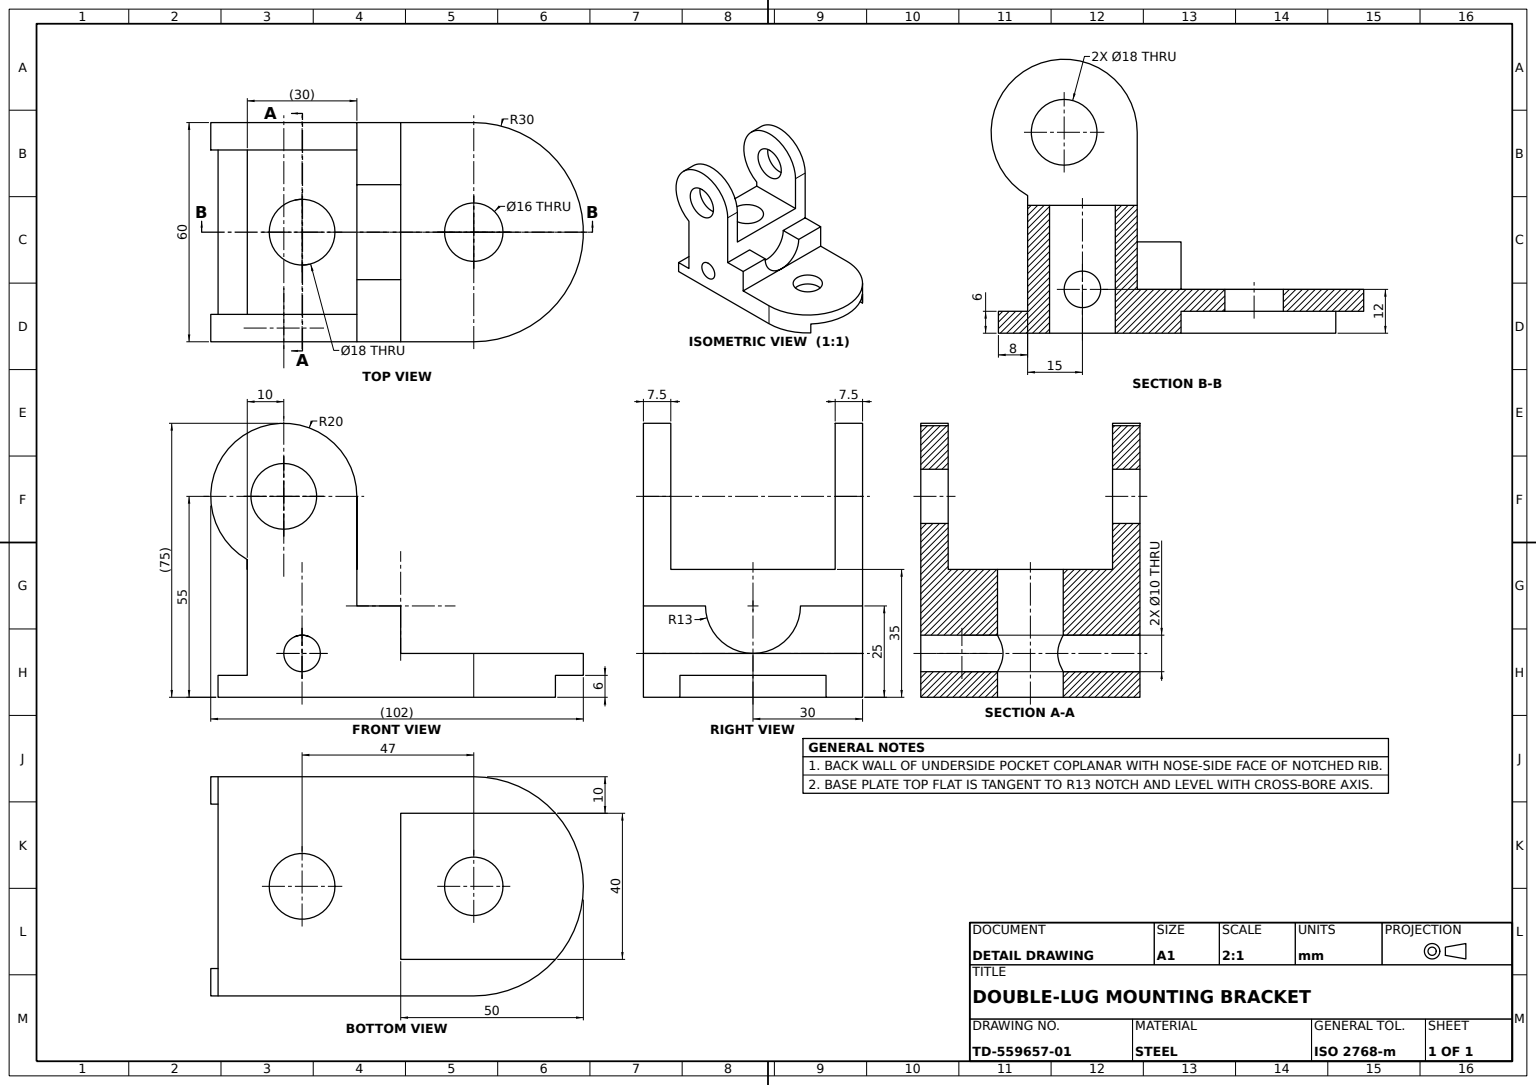
ISO-10303-21;
HEADER;
FILE_DESCRIPTION((''),'2;1');
FILE_NAME('','',(''),(''),'','','');
FILE_SCHEMA(('AUTOMOTIVE_DESIGN'));
ENDSEC;
DATA;
#1=APPLICATION_CONTEXT('');
#2=PRODUCT_CONTEXT('',#1,'mechanical');
#3=PRODUCT('','','',(#2));
#4=PRODUCT_DEFINITION_FORMATION('','',#3);
#5=PRODUCT_DEFINITION_CONTEXT('',#1,'design');
#6=PRODUCT_DEFINITION('','',#4,#5);
#7=PRODUCT_DEFINITION_SHAPE('','',#6);
#8=(LENGTH_UNIT()NAMED_UNIT(*)SI_UNIT(.MILLI.,.METRE.));
#9=(NAMED_UNIT(*)PLANE_ANGLE_UNIT()SI_UNIT($,.RADIAN.));
#10=(NAMED_UNIT(*)SI_UNIT($,.STERADIAN.)SOLID_ANGLE_UNIT());
#11=UNCERTAINTY_MEASURE_WITH_UNIT(LENGTH_MEASURE(0.005),#8,'distance_accuracy_value','');
#12=(GEOMETRIC_REPRESENTATION_CONTEXT(3)GLOBAL_UNCERTAINTY_ASSIGNED_CONTEXT((#11))GLOBAL_UNIT_ASSIGNED_CONTEXT((#8,#9,#10))REPRESENTATION_CONTEXT('',''));
#13=CARTESIAN_POINT('',(12.,0.,12.));
#14=VERTEX_POINT('',#13);
#15=CARTESIAN_POINT('',(20.,0.,12.));
#16=DIRECTION('',(0.,0.,-1.));
#17=DIRECTION('',(-1.,0.,0.));
#18=AXIS2_PLACEMENT_3D('',#15,#16,#17);
#19=CIRCLE('',#18,8.);
#20=EDGE_CURVE('',#14,#14,#19,.T.);
#21=ORIENTED_EDGE('',*,*,#20,.T.);
#22=EDGE_LOOP('',(#21));
#23=FACE_BOUND('',#22,.T.);
#24=CARTESIAN_POINT('',(0.,-30.,12.));
#25=VERTEX_POINT('',#24);
#26=CARTESIAN_POINT('',(0.,0.,12.));
#27=VERTEX_POINT('',#26);
#28=DIRECTION('',(0.,1.,0.));
#29=VECTOR('',#28,1000.);
#30=LINE('',#24,#29);
#31=EDGE_CURVE('',#25,#27,#30,.T.);
#32=ORIENTED_EDGE('',*,*,#31,.F.);
#33=CARTESIAN_POINT('',(20.,-30.,12.));
#34=VERTEX_POINT('',#33);
#35=CARTESIAN_POINT('',(-50.,-30.,12.));
#36=DIRECTION('',(1.,0.,0.));
#37=VECTOR('',#36,1000.);
#38=LINE('',#35,#37);
#39=EDGE_CURVE('',#25,#34,#38,.T.);
#40=ORIENTED_EDGE('',*,*,#39,.T.);
#41=CARTESIAN_POINT('',(20.,30.,12.));
#42=VERTEX_POINT('',#41);
#43=DIRECTION('',(0.,0.,1.));
#44=AXIS2_PLACEMENT_3D('',#15,#43,#36);
#45=CIRCLE('',#44,30.);
#46=EDGE_CURVE('',#34,#42,#45,.T.);
#47=ORIENTED_EDGE('',*,*,#46,.T.);
#48=CARTESIAN_POINT('',(0.,30.,12.));
#49=VERTEX_POINT('',#48);
#50=VECTOR('',#17,1000.);
#51=LINE('',#41,#50);
#52=EDGE_CURVE('',#42,#49,#51,.T.);
#53=ORIENTED_EDGE('',*,*,#52,.T.);
#54=EDGE_CURVE('',#27,#49,#30,.T.);
#55=ORIENTED_EDGE('',*,*,#54,.F.);
#56=EDGE_LOOP('',(#32,#40,#47,#53,#55));
#57=FACE_BOUND('',#56,.T.);
#58=PLANE('',#44);
#59=ADVANCED_FACE('',(#23,#57),#58,.T.);
#60=CARTESIAN_POINT('',(-12.,-30.,55.));
#61=VERTEX_POINT('',#60);
#62=CARTESIAN_POINT('',(-12.,-22.5,55.));
#63=VERTEX_POINT('',#62);
#64=LINE('',#60,#29);
#65=EDGE_CURVE('',#61,#63,#64,.T.);
#66=ORIENTED_EDGE('',*,*,#65,.T.);
#67=CARTESIAN_POINT('',(-42.,-22.5,37.679492));
#68=VERTEX_POINT('',#67);
#69=CARTESIAN_POINT('',(-32.,-22.5,55.));
#70=DIRECTION('',(0.,-1.,0.));
#71=AXIS2_PLACEMENT_3D('',#69,#70,#36);
#72=CIRCLE('',#71,20.);
#73=EDGE_CURVE('',#68,#63,#72,.F.);
#74=ORIENTED_EDGE('',*,*,#73,.F.);
#75=CARTESIAN_POINT('',(-42.,-30.,37.679492));
#76=VERTEX_POINT('',#75);
#77=LINE('',#75,#29);
#78=EDGE_CURVE('',#76,#68,#77,.T.);
#79=ORIENTED_EDGE('',*,*,#78,.F.);
#80=CARTESIAN_POINT('',(-32.,-30.,55.));
#81=AXIS2_PLACEMENT_3D('',#80,#28,#36);
#82=CIRCLE('',#81,20.);
#83=EDGE_CURVE('',#76,#61,#82,.T.);
#84=ORIENTED_EDGE('',*,*,#83,.T.);
#85=EDGE_LOOP('',(#66,#74,#79,#84));
#86=FACE_BOUND('',#85,.T.);
#87=AXIS2_PLACEMENT_3D('',#80,#28,#43);
#88=CYLINDRICAL_SURFACE('',#87,20.);
#89=ADVANCED_FACE('',(#86),#88,.T.);
#90=CARTESIAN_POINT('',(-32.,30.,64.));
#91=VERTEX_POINT('',#90);
#92=CARTESIAN_POINT('',(-32.,30.,55.));
#93=AXIS2_PLACEMENT_3D('',#92,#28,#43);
#94=CIRCLE('',#93,9.);
#95=EDGE_CURVE('',#91,#91,#94,.T.);
#96=ORIENTED_EDGE('',*,*,#95,.F.);
#97=EDGE_LOOP('',(#96));
#98=FACE_BOUND('',#97,.T.);
#99=CARTESIAN_POINT('',(-27.,30.,17.));
#100=VERTEX_POINT('',#99);
#101=CARTESIAN_POINT('',(-27.,30.,12.));
#102=AXIS2_PLACEMENT_3D('',#101,#28,#43);
#103=CIRCLE('',#102,5.);
#104=EDGE_CURVE('',#100,#100,#103,.T.);
#105=ORIENTED_EDGE('',*,*,#104,.F.);
#106=EDGE_LOOP('',(#105));
#107=FACE_BOUND('',#106,.T.);
#108=CARTESIAN_POINT('',(-12.,30.,55.));
#109=VERTEX_POINT('',#108);
#110=CARTESIAN_POINT('',(-12.,30.,25.));
#111=VERTEX_POINT('',#110);
#112=VECTOR('',#16,1000.);
#113=LINE('',#108,#112);
#114=EDGE_CURVE('',#109,#111,#113,.T.);
#115=ORIENTED_EDGE('',*,*,#114,.T.);
#116=CARTESIAN_POINT('',(0.,30.,25.));
#117=VERTEX_POINT('',#116);
#118=LINE('',#110,#37);
#119=EDGE_CURVE('',#111,#117,#118,.T.);
#120=ORIENTED_EDGE('',*,*,#119,.T.);
#121=LINE('',#116,#112);
#122=EDGE_CURVE('',#117,#49,#121,.T.);
#123=ORIENTED_EDGE('',*,*,#122,.T.);
#124=ORIENTED_EDGE('',*,*,#52,.F.);
#125=CARTESIAN_POINT('',(20.,30.,0.));
#126=VERTEX_POINT('',#125);
#127=LINE('',#41,#112);
#128=EDGE_CURVE('',#42,#126,#127,.T.);
#129=ORIENTED_EDGE('',*,*,#128,.T.);
#130=CARTESIAN_POINT('',(-50.,30.,0.));
#131=VERTEX_POINT('',#130);
#132=LINE('',#125,#50);
#133=EDGE_CURVE('',#126,#131,#132,.T.);
#134=ORIENTED_EDGE('',*,*,#133,.T.);
#135=CARTESIAN_POINT('',(-50.,30.,6.));
#136=VERTEX_POINT('',#135);
#137=CARTESIAN_POINT('',(-50.,30.,12.));
#138=LINE('',#137,#112);
#139=EDGE_CURVE('',#136,#131,#138,.T.);
#140=ORIENTED_EDGE('',*,*,#139,.F.);
#141=CARTESIAN_POINT('',(-42.,30.,6.));
#142=VERTEX_POINT('',#141);
#143=CARTESIAN_POINT('',(-32.,30.,6.));
#144=LINE('',#143,#50);
#145=EDGE_CURVE('',#142,#136,#144,.T.);
#146=ORIENTED_EDGE('',*,*,#145,.F.);
#147=CARTESIAN_POINT('',(-42.,30.,37.679492));
#148=VERTEX_POINT('',#147);
#149=VECTOR('',#43,1000.);
#150=LINE('',#141,#149);
#151=EDGE_CURVE('',#142,#148,#150,.T.);
#152=ORIENTED_EDGE('',*,*,#151,.T.);
#153=AXIS2_PLACEMENT_3D('',#92,#28,#36);
#154=CIRCLE('',#153,20.);
#155=EDGE_CURVE('',#148,#109,#154,.T.);
#156=ORIENTED_EDGE('',*,*,#155,.T.);
#157=EDGE_LOOP('',(#115,#120,#123,#124,#129,#134,#140,#146,#152,#156));
#158=FACE_BOUND('',#157,.T.);
#159=PLANE('',#93);
#160=ADVANCED_FACE('',(#98,#107,#158),#159,.T.);
#161=CARTESIAN_POINT('',(-32.,22.5,64.));
#162=VERTEX_POINT('',#161);
#163=CARTESIAN_POINT('',(-32.,22.5,55.));
#164=AXIS2_PLACEMENT_3D('',#163,#28,#43);
#165=CIRCLE('',#164,9.);
#166=EDGE_CURVE('',#162,#162,#165,.F.);
#167=ORIENTED_EDGE('',*,*,#166,.F.);
#168=EDGE_LOOP('',(#167));
#169=FACE_BOUND('',#168,.T.);
#170=CARTESIAN_POINT('',(-42.,22.5,37.679492));
#171=VERTEX_POINT('',#170);
#172=CARTESIAN_POINT('',(-42.,22.5,35.));
#173=VERTEX_POINT('',#172);
#174=CARTESIAN_POINT('',(-42.,22.5,6.));
#175=LINE('',#174,#112);
#176=EDGE_CURVE('',#171,#173,#175,.T.);
#177=ORIENTED_EDGE('',*,*,#176,.T.);
#178=CARTESIAN_POINT('',(-12.,22.5,35.));
#179=VERTEX_POINT('',#178);
#180=CARTESIAN_POINT('',(-53.645444,22.5,35.));
#181=LINE('',#180,#37);
#182=EDGE_CURVE('',#179,#173,#181,.F.);
#183=ORIENTED_EDGE('',*,*,#182,.F.);
#184=CARTESIAN_POINT('',(-12.,22.5,55.));
#185=VERTEX_POINT('',#184);
#186=LINE('',#184,#149);
#187=EDGE_CURVE('',#179,#185,#186,.T.);
#188=ORIENTED_EDGE('',*,*,#187,.T.);
#189=CIRCLE('',#164,20.);
#190=EDGE_CURVE('',#185,#171,#189,.F.);
#191=ORIENTED_EDGE('',*,*,#190,.T.);
#192=EDGE_LOOP('',(#177,#183,#188,#191));
#193=FACE_BOUND('',#192,.T.);
#194=CARTESIAN_POINT('',(-53.645444,22.5,102.));
#195=AXIS2_PLACEMENT_3D('',#194,#28,#43);
#196=PLANE('',#195);
#197=ADVANCED_FACE('',(#169,#193),#196,.F.);
#198=ORIENTED_EDGE('',*,*,#95,.T.);
#199=EDGE_LOOP('',(#198));
#200=FACE_BOUND('',#199,.T.);
#201=ORIENTED_EDGE('',*,*,#166,.T.);
#202=EDGE_LOOP('',(#201));
#203=FACE_BOUND('',#202,.T.);
#204=CYLINDRICAL_SURFACE('',#87,9.);
#205=ADVANCED_FACE('',(#200,#203),#204,.F.);
#206=CARTESIAN_POINT('',(-12.,13.,25.));
#207=VERTEX_POINT('',#206);
#208=CARTESIAN_POINT('',(0.,13.,25.));
#209=VERTEX_POINT('',#208);
#210=CARTESIAN_POINT('',(30.,13.,25.));
#211=LINE('',#210,#50);
#212=EDGE_CURVE('',#207,#209,#211,.F.);
#213=ORIENTED_EDGE('',*,*,#212,.T.);
#214=CARTESIAN_POINT('',(0.,-30.,25.));
#215=LINE('',#214,#29);
#216=EDGE_CURVE('',#209,#117,#215,.T.);
#217=ORIENTED_EDGE('',*,*,#216,.T.);
#218=ORIENTED_EDGE('',*,*,#119,.F.);
#219=CARTESIAN_POINT('',(-12.,-30.,25.));
#220=LINE('',#219,#29);
#221=EDGE_CURVE('',#207,#111,#220,.T.);
#222=ORIENTED_EDGE('',*,*,#221,.F.);
#223=EDGE_LOOP('',(#213,#217,#218,#222));
#224=FACE_BOUND('',#223,.T.);
#225=AXIS2_PLACEMENT_3D('',#219,#43,#36);
#226=PLANE('',#225);
#227=ADVANCED_FACE('',(#224),#226,.T.);
#228=ORIENTED_EDGE('',*,*,#187,.F.);
#229=CARTESIAN_POINT('',(-12.,-22.5,35.));
#230=VERTEX_POINT('',#229);
#231=CARTESIAN_POINT('',(-12.,-30.,35.));
#232=LINE('',#231,#29);
#233=EDGE_CURVE('',#230,#179,#232,.T.);
#234=ORIENTED_EDGE('',*,*,#233,.F.);
#235=LINE('',#62,#112);
#236=EDGE_CURVE('',#63,#230,#235,.T.);
#237=ORIENTED_EDGE('',*,*,#236,.F.);
#238=ORIENTED_EDGE('',*,*,#65,.F.);
#239=VERTEX_POINT('',#219);
#240=LINE('',#60,#112);
#241=EDGE_CURVE('',#61,#239,#240,.T.);
#242=ORIENTED_EDGE('',*,*,#241,.T.);
#243=CARTESIAN_POINT('',(-12.,-13.,25.));
#244=VERTEX_POINT('',#243);
#245=EDGE_CURVE('',#239,#244,#220,.T.);
#246=ORIENTED_EDGE('',*,*,#245,.T.);
#247=CARTESIAN_POINT('',(-12.,0.,25.));
#248=AXIS2_PLACEMENT_3D('',#247,#36,#28);
#249=CIRCLE('',#248,13.);
#250=EDGE_CURVE('',#244,#207,#249,.T.);
#251=ORIENTED_EDGE('',*,*,#250,.T.);
#252=ORIENTED_EDGE('',*,*,#221,.T.);
#253=ORIENTED_EDGE('',*,*,#114,.F.);
#254=EDGE_CURVE('',#185,#109,#64,.T.);
#255=ORIENTED_EDGE('',*,*,#254,.F.);
#256=EDGE_LOOP('',(#228,#234,#237,#238,#242,#246,#251,#252,#253,#255));
#257=FACE_BOUND('',#256,.T.);
#258=AXIS2_PLACEMENT_3D('',#60,#36,#16);
#259=PLANE('',#258);
#260=ADVANCED_FACE('',(#257),#259,.T.);
#261=CARTESIAN_POINT('',(-27.,-9.,17.));
#262=VERTEX_POINT('',#261);
#263=CARTESIAN_POINT('',(-24.993316,-8.841607,16.722393));
#264=CARTESIAN_POINT('',(-27.000875,-9.079032,17.138457));
#265=CARTESIAN_POINT('',(-29.003185,-8.842266,16.723778));
#266=CARTESIAN_POINT('',(-30.626784,-8.28236,15.616044));
#267=CARTESIAN_POINT('',(-31.718659,-7.680388,14.00946));
#268=CARTESIAN_POINT('',(-32.138945,-7.385853,12.00846));
#269=CARTESIAN_POINT('',(-31.725524,-7.676113,10.004354));
#270=CARTESIAN_POINT('',(-30.631385,-8.280339,8.388065));
#271=CARTESIAN_POINT('',(-29.013325,-8.83947,7.281492));
#272=CARTESIAN_POINT('',(-27.015518,-9.079002,6.861607));
#273=CARTESIAN_POINT('',(-25.003645,-8.844464,7.272186));
#274=CARTESIAN_POINT('',(-23.376847,-8.284028,8.380154));
#275=CARTESIAN_POINT('',(-22.282,-7.680923,9.98776));
#276=CARTESIAN_POINT('',(-21.860693,-7.38556,11.99248));
#277=CARTESIAN_POINT('',(-22.275262,-7.676746,13.998416));
#278=CARTESIAN_POINT('',(-23.372652,-8.28217,15.616187));
#279=B_SPLINE_CURVE_WITH_KNOTS('',3,(#263,#264,#265,#266,#267,#268,#269,#270,#271,#272,#273,#274,#275,#276,#277,#278,#263,#264,#265),.UNSPECIFIED.,.T.,.F.,(1,1,1,1,1,1,1,1,1,1,1,1,1,1,1,1,1,1,1,1,1,1,1),(-0.005985549,-0.003990366,-0.001995183,0.,0.001995183,0.003990366,0.005985549,0.007980732,0.009975915,0.011971098,0.013966282,0.015961465,0.017956648,0.019951831,0.021947014,0.023942197,0.02593738,0.027932563,0.029927746,0.031922929,0.033918112,0.035913295,0.037908478),.UNSPECIFIED.);
#280=EDGE_CURVE('',#262,#262,#279,.T.);
#281=ORIENTED_EDGE('',*,*,#280,.F.);
#282=EDGE_LOOP('',(#281));
#283=FACE_BOUND('',#282,.T.);
#284=CARTESIAN_POINT('',(-27.,-30.,17.));
#285=VERTEX_POINT('',#284);
#286=CARTESIAN_POINT('',(-27.,-30.,12.));
#287=AXIS2_PLACEMENT_3D('',#286,#28,#43);
#288=CIRCLE('',#287,5.);
#289=EDGE_CURVE('',#285,#285,#288,.T.);
#290=ORIENTED_EDGE('',*,*,#289,.F.);
#291=EDGE_LOOP('',(#290));
#292=FACE_BOUND('',#291,.T.);
#293=CYLINDRICAL_SURFACE('',#287,5.);
#294=ADVANCED_FACE('',(#283,#292),#293,.F.);
#295=ORIENTED_EDGE('',*,*,#254,.T.);
#296=ORIENTED_EDGE('',*,*,#155,.F.);
#297=EDGE_CURVE('',#171,#148,#77,.T.);
#298=ORIENTED_EDGE('',*,*,#297,.F.);
#299=ORIENTED_EDGE('',*,*,#190,.F.);
#300=EDGE_LOOP('',(#295,#296,#298,#299));
#301=FACE_BOUND('',#300,.T.);
#302=ADVANCED_FACE('',(#301),#88,.T.);
#303=ORIENTED_EDGE('',*,*,#250,.F.);
#304=CARTESIAN_POINT('',(0.,-13.,25.));
#305=VERTEX_POINT('',#304);
#306=CARTESIAN_POINT('',(30.,-13.,25.));
#307=LINE('',#306,#50);
#308=EDGE_CURVE('',#305,#244,#307,.T.);
#309=ORIENTED_EDGE('',*,*,#308,.F.);
#310=CARTESIAN_POINT('',(0.,0.,25.));
#311=AXIS2_PLACEMENT_3D('',#310,#36,#16);
#312=CIRCLE('',#311,13.);
#313=EDGE_CURVE('',#27,#305,#312,.F.);
#314=ORIENTED_EDGE('',*,*,#313,.F.);
#315=EDGE_CURVE('',#209,#27,#312,.F.);
#316=ORIENTED_EDGE('',*,*,#315,.F.);
#317=ORIENTED_EDGE('',*,*,#212,.F.);
#318=EDGE_LOOP('',(#303,#309,#314,#316,#317));
#319=FACE_BOUND('',#318,.T.);
#320=CARTESIAN_POINT('',(30.,0.,25.));
#321=AXIS2_PLACEMENT_3D('',#320,#17,#43);
#322=CYLINDRICAL_SURFACE('',#321,13.);
#323=ADVANCED_FACE('',(#319),#322,.F.);
#324=ORIENTED_EDGE('',*,*,#280,.T.);
#325=EDGE_LOOP('',(#324));
#326=FACE_BOUND('',#325,.T.);
#327=CARTESIAN_POINT('',(-36.,0.,35.));
#328=VERTEX_POINT('',#327);
#329=CARTESIAN_POINT('',(-27.,0.,35.));
#330=AXIS2_PLACEMENT_3D('',#329,#16,#17);
#331=CIRCLE('',#330,9.);
#332=EDGE_CURVE('',#328,#328,#331,.T.);
#333=ORIENTED_EDGE('',*,*,#332,.F.);
#334=EDGE_LOOP('',(#333));
#335=FACE_BOUND('',#334,.T.);
#336=CARTESIAN_POINT('',(-18.,0.,0.));
#337=VERTEX_POINT('',#336);
#338=CARTESIAN_POINT('',(-27.,0.,0.));
#339=AXIS2_PLACEMENT_3D('',#338,#43,#36);
#340=CIRCLE('',#339,9.);
#341=EDGE_CURVE('',#337,#337,#340,.T.);
#342=ORIENTED_EDGE('',*,*,#341,.F.);
#343=EDGE_LOOP('',(#342));
#344=FACE_BOUND('',#343,.T.);
#345=CARTESIAN_POINT('',(-27.,9.,17.));
#346=VERTEX_POINT('',#345);
#347=CARTESIAN_POINT('',(-29.006684,8.841607,16.722393));
#348=CARTESIAN_POINT('',(-26.999125,9.079032,17.138457));
#349=CARTESIAN_POINT('',(-24.996815,8.842266,16.723778));
#350=CARTESIAN_POINT('',(-23.373216,8.28236,15.616044));
#351=CARTESIAN_POINT('',(-22.281341,7.680388,14.00946));
#352=CARTESIAN_POINT('',(-21.861055,7.385853,12.00846));
#353=CARTESIAN_POINT('',(-22.274476,7.676113,10.004354));
#354=CARTESIAN_POINT('',(-23.368615,8.280339,8.388065));
#355=CARTESIAN_POINT('',(-24.986675,8.83947,7.281492));
#356=CARTESIAN_POINT('',(-26.984482,9.079002,6.861607));
#357=CARTESIAN_POINT('',(-28.996355,8.844464,7.272186));
#358=CARTESIAN_POINT('',(-30.623153,8.284028,8.380154));
#359=CARTESIAN_POINT('',(-31.718,7.680923,9.98776));
#360=CARTESIAN_POINT('',(-32.139307,7.38556,11.99248));
#361=CARTESIAN_POINT('',(-31.724738,7.676746,13.998416));
#362=CARTESIAN_POINT('',(-30.627348,8.28217,15.616187));
#363=B_SPLINE_CURVE_WITH_KNOTS('',3,(#347,#348,#349,#350,#351,#352,#353,#354,#355,#356,#357,#358,#359,#360,#361,#362,#347,#348,#349),.UNSPECIFIED.,.T.,.F.,(1,1,1,1,1,1,1,1,1,1,1,1,1,1,1,1,1,1,1,1,1,1,1),(-0.005985549,-0.003990366,-0.001995183,0.,0.001995183,0.003990366,0.005985549,0.007980732,0.009975915,0.011971098,0.013966282,0.015961465,0.017956648,0.019951831,0.021947014,0.023942197,0.02593738,0.027932563,0.029927746,0.031922929,0.033918112,0.035913295,0.037908478),.UNSPECIFIED.);
#364=EDGE_CURVE('',#346,#346,#363,.T.);
#365=ORIENTED_EDGE('',*,*,#364,.T.);
#366=EDGE_LOOP('',(#365));
#367=FACE_BOUND('',#366,.T.);
#368=CYLINDRICAL_SURFACE('',#330,9.);
#369=ADVANCED_FACE('',(#326,#335,#344,#367),#368,.F.);
#370=ORIENTED_EDGE('',*,*,#364,.F.);
#371=EDGE_LOOP('',(#370));
#372=FACE_BOUND('',#371,.T.);
#373=ORIENTED_EDGE('',*,*,#104,.T.);
#374=EDGE_LOOP('',(#373));
#375=FACE_BOUND('',#374,.T.);
#376=ADVANCED_FACE('',(#372,#375),#293,.F.);
#377=CARTESIAN_POINT('',(42.36068,20.,6.));
#378=VERTEX_POINT('',#377);
#379=CARTESIAN_POINT('',(42.36068,20.,0.));
#380=VERTEX_POINT('',#379);
#381=CARTESIAN_POINT('',(42.36068,20.,12.));
#382=LINE('',#381,#112);
#383=EDGE_CURVE('',#378,#380,#382,.T.);
#384=ORIENTED_EDGE('',*,*,#383,.F.);
#385=CARTESIAN_POINT('',(0.,20.,6.));
#386=VERTEX_POINT('',#385);
#387=CARTESIAN_POINT('',(60.,20.,6.));
#388=LINE('',#387,#50);
#389=EDGE_CURVE('',#386,#378,#388,.F.);
#390=ORIENTED_EDGE('',*,*,#389,.F.);
#391=CARTESIAN_POINT('',(0.,20.,0.));
#392=VERTEX_POINT('',#391);
#393=LINE('',#391,#149);
#394=EDGE_CURVE('',#386,#392,#393,.F.);
#395=ORIENTED_EDGE('',*,*,#394,.T.);
#396=CARTESIAN_POINT('',(60.,20.,0.));
#397=LINE('',#396,#50);
#398=EDGE_CURVE('',#380,#392,#397,.T.);
#399=ORIENTED_EDGE('',*,*,#398,.F.);
#400=EDGE_LOOP('',(#384,#390,#395,#399));
#401=FACE_BOUND('',#400,.T.);
#402=AXIS2_PLACEMENT_3D('',#396,#28,#17);
#403=PLANE('',#402);
#404=ADVANCED_FACE('',(#401),#403,.F.);
#405=ORIENTED_EDGE('',*,*,#54,.T.);
#406=ORIENTED_EDGE('',*,*,#122,.F.);
#407=ORIENTED_EDGE('',*,*,#216,.F.);
#408=ORIENTED_EDGE('',*,*,#315,.T.);
#409=EDGE_LOOP('',(#405,#406,#407,#408));
#410=FACE_BOUND('',#409,.T.);
#411=AXIS2_PLACEMENT_3D('',#214,#36,#16);
#412=PLANE('',#411);
#413=ADVANCED_FACE('',(#410),#412,.T.);
#414=CARTESIAN_POINT('',(-50.,-30.,0.));
#415=VERTEX_POINT('',#414);
#416=VECTOR('',#70,1000.);
#417=LINE('',#130,#416);
#418=EDGE_CURVE('',#131,#415,#417,.T.);
#419=ORIENTED_EDGE('',*,*,#418,.T.);
#420=CARTESIAN_POINT('',(-50.,-30.,6.));
#421=VERTEX_POINT('',#420);
#422=LINE('',#35,#112);
#423=EDGE_CURVE('',#421,#415,#422,.T.);
#424=ORIENTED_EDGE('',*,*,#423,.F.);
#425=CARTESIAN_POINT('',(-50.,-32.,6.));
#426=LINE('',#425,#29);
#427=EDGE_CURVE('',#421,#136,#426,.T.);
#428=ORIENTED_EDGE('',*,*,#427,.T.);
#429=ORIENTED_EDGE('',*,*,#139,.T.);
#430=EDGE_LOOP('',(#419,#424,#428,#429));
#431=FACE_BOUND('',#430,.T.);
#432=AXIS2_PLACEMENT_3D('',#137,#36,#16);
#433=PLANE('',#432);
#434=ADVANCED_FACE('',(#431),#433,.F.);
#435=CARTESIAN_POINT('',(-42.,-22.5,35.));
#436=VERTEX_POINT('',#435);
#437=CARTESIAN_POINT('',(-42.,-30.,35.));
#438=LINE('',#437,#416);
#439=EDGE_CURVE('',#173,#436,#438,.T.);
#440=ORIENTED_EDGE('',*,*,#439,.F.);
#441=ORIENTED_EDGE('',*,*,#176,.F.);
#442=ORIENTED_EDGE('',*,*,#297,.T.);
#443=ORIENTED_EDGE('',*,*,#151,.F.);
#444=CARTESIAN_POINT('',(-42.,-30.,6.));
#445=VERTEX_POINT('',#444);
#446=CARTESIAN_POINT('',(-42.,-32.,6.));
#447=LINE('',#446,#29);
#448=EDGE_CURVE('',#445,#142,#447,.T.);
#449=ORIENTED_EDGE('',*,*,#448,.F.);
#450=LINE('',#444,#149);
#451=EDGE_CURVE('',#445,#76,#450,.T.);
#452=ORIENTED_EDGE('',*,*,#451,.T.);
#453=ORIENTED_EDGE('',*,*,#78,.T.);
#454=CARTESIAN_POINT('',(-42.,-22.5,6.));
#455=LINE('',#454,#149);
#456=EDGE_CURVE('',#436,#68,#455,.T.);
#457=ORIENTED_EDGE('',*,*,#456,.F.);
#458=EDGE_LOOP('',(#440,#441,#442,#443,#449,#452,#453,#457));
#459=FACE_BOUND('',#458,.T.);
#460=AXIS2_PLACEMENT_3D('',#444,#17,#43);
#461=PLANE('',#460);
#462=ADVANCED_FACE('',(#459),#461,.T.);
#463=ORIENTED_EDGE('',*,*,#394,.F.);
#464=CARTESIAN_POINT('',(0.,-20.,6.));
#465=VERTEX_POINT('',#464);
#466=LINE('',#385,#416);
#467=EDGE_CURVE('',#465,#386,#466,.F.);
#468=ORIENTED_EDGE('',*,*,#467,.F.);
#469=CARTESIAN_POINT('',(0.,-20.,0.));
#470=VERTEX_POINT('',#469);
#471=LINE('',#469,#149);
#472=EDGE_CURVE('',#465,#470,#471,.F.);
#473=ORIENTED_EDGE('',*,*,#472,.T.);
#474=LINE('',#391,#416);
#475=EDGE_CURVE('',#392,#470,#474,.T.);
#476=ORIENTED_EDGE('',*,*,#475,.F.);
#477=EDGE_LOOP('',(#463,#468,#473,#476));
#478=FACE_BOUND('',#477,.T.);
#479=AXIS2_PLACEMENT_3D('',#391,#17,#43);
#480=PLANE('',#479);
#481=ADVANCED_FACE('',(#478),#480,.F.);
#482=CARTESIAN_POINT('',(-23.,-22.5,55.));
#483=VERTEX_POINT('',#482);
#484=CIRCLE('',#71,9.);
#485=EDGE_CURVE('',#483,#483,#484,.F.);
#486=ORIENTED_EDGE('',*,*,#485,.T.);
#487=EDGE_LOOP('',(#486));
#488=FACE_BOUND('',#487,.T.);
#489=CARTESIAN_POINT('',(-32.,-30.,64.));
#490=VERTEX_POINT('',#489);
#491=CIRCLE('',#87,9.);
#492=EDGE_CURVE('',#490,#490,#491,.T.);
#493=ORIENTED_EDGE('',*,*,#492,.F.);
#494=EDGE_LOOP('',(#493));
#495=FACE_BOUND('',#494,.T.);
#496=ADVANCED_FACE('',(#488,#495),#204,.F.);
#497=CARTESIAN_POINT('',(28.,0.,6.));
#498=VERTEX_POINT('',#497);
#499=CARTESIAN_POINT('',(20.,0.,6.));
#500=AXIS2_PLACEMENT_3D('',#499,#43,#36);
#501=CIRCLE('',#500,8.);
#502=EDGE_CURVE('',#498,#498,#501,.T.);
#503=ORIENTED_EDGE('',*,*,#502,.F.);
#504=EDGE_LOOP('',(#503));
#505=FACE_BOUND('',#504,.T.);
#506=ORIENTED_EDGE('',*,*,#20,.F.);
#507=EDGE_LOOP('',(#506));
#508=FACE_BOUND('',#507,.T.);
#509=CYLINDRICAL_SURFACE('',#18,8.);
#510=ADVANCED_FACE('',(#505,#508),#509,.F.);
#511=ORIENTED_EDGE('',*,*,#289,.T.);
#512=EDGE_LOOP('',(#511));
#513=FACE_BOUND('',#512,.T.);
#514=ORIENTED_EDGE('',*,*,#492,.T.);
#515=EDGE_LOOP('',(#514));
#516=FACE_BOUND('',#515,.T.);
#517=VERTEX_POINT('',#214);
#518=LINE('',#219,#37);
#519=EDGE_CURVE('',#239,#517,#518,.T.);
#520=ORIENTED_EDGE('',*,*,#519,.F.);
#521=ORIENTED_EDGE('',*,*,#241,.F.);
#522=ORIENTED_EDGE('',*,*,#83,.F.);
#523=ORIENTED_EDGE('',*,*,#451,.F.);
#524=CARTESIAN_POINT('',(-32.,-30.,6.));
#525=LINE('',#524,#50);
#526=EDGE_CURVE('',#445,#421,#525,.T.);
#527=ORIENTED_EDGE('',*,*,#526,.T.);
#528=ORIENTED_EDGE('',*,*,#423,.T.);
#529=CARTESIAN_POINT('',(20.,-30.,0.));
#530=VERTEX_POINT('',#529);
#531=LINE('',#414,#37);
#532=EDGE_CURVE('',#415,#530,#531,.T.);
#533=ORIENTED_EDGE('',*,*,#532,.T.);
#534=LINE('',#33,#112);
#535=EDGE_CURVE('',#34,#530,#534,.T.);
#536=ORIENTED_EDGE('',*,*,#535,.F.);
#537=ORIENTED_EDGE('',*,*,#39,.F.);
#538=LINE('',#214,#112);
#539=EDGE_CURVE('',#517,#25,#538,.T.);
#540=ORIENTED_EDGE('',*,*,#539,.F.);
#541=EDGE_LOOP('',(#520,#521,#522,#523,#527,#528,#533,#536,#537,#540));
#542=FACE_BOUND('',#541,.T.);
#543=PLANE('',#87);
#544=ADVANCED_FACE('',(#513,#516,#542),#543,.F.);
#545=CARTESIAN_POINT('',(42.36068,-20.,0.));
#546=VERTEX_POINT('',#545);
#547=CARTESIAN_POINT('',(42.36068,-20.,6.));
#548=VERTEX_POINT('',#547);
#549=CARTESIAN_POINT('',(42.36068,-20.,12.));
#550=LINE('',#549,#112);
#551=EDGE_CURVE('',#546,#548,#550,.F.);
#552=ORIENTED_EDGE('',*,*,#551,.F.);
#553=LINE('',#469,#37);
#554=EDGE_CURVE('',#470,#546,#553,.T.);
#555=ORIENTED_EDGE('',*,*,#554,.F.);
#556=ORIENTED_EDGE('',*,*,#472,.F.);
#557=LINE('',#464,#37);
#558=EDGE_CURVE('',#548,#465,#557,.F.);
#559=ORIENTED_EDGE('',*,*,#558,.F.);
#560=EDGE_LOOP('',(#552,#555,#556,#559));
#561=FACE_BOUND('',#560,.T.);
#562=AXIS2_PLACEMENT_3D('',#469,#70,#36);
#563=PLANE('',#562);
#564=ADVANCED_FACE('',(#561),#563,.F.);
#565=ORIENTED_EDGE('',*,*,#341,.T.);
#566=EDGE_LOOP('',(#565));
#567=FACE_BOUND('',#566,.T.);
#568=ORIENTED_EDGE('',*,*,#554,.T.);
#569=CARTESIAN_POINT('',(20.,0.,0.));
#570=AXIS2_PLACEMENT_3D('',#569,#43,#36);
#571=CIRCLE('',#570,30.);
#572=EDGE_CURVE('',#530,#546,#571,.T.);
#573=ORIENTED_EDGE('',*,*,#572,.F.);
#574=ORIENTED_EDGE('',*,*,#532,.F.);
#575=ORIENTED_EDGE('',*,*,#418,.F.);
#576=ORIENTED_EDGE('',*,*,#133,.F.);
#577=EDGE_CURVE('',#380,#126,#571,.T.);
#578=ORIENTED_EDGE('',*,*,#577,.F.);
#579=ORIENTED_EDGE('',*,*,#398,.T.);
#580=ORIENTED_EDGE('',*,*,#475,.T.);
#581=EDGE_LOOP('',(#568,#573,#574,#575,#576,#578,#579,#580));
#582=FACE_BOUND('',#581,.T.);
#583=PLANE('',#570);
#584=ADVANCED_FACE('',(#567,#582),#583,.F.);
#585=ORIENTED_EDGE('',*,*,#73,.T.);
#586=ORIENTED_EDGE('',*,*,#236,.T.);
#587=CARTESIAN_POINT('',(-11.955925,-22.5,35.));
#588=LINE('',#587,#50);
#589=EDGE_CURVE('',#436,#230,#588,.F.);
#590=ORIENTED_EDGE('',*,*,#589,.F.);
#591=ORIENTED_EDGE('',*,*,#456,.T.);
#592=EDGE_LOOP('',(#585,#586,#590,#591));
#593=FACE_BOUND('',#592,.T.);
#594=ORIENTED_EDGE('',*,*,#485,.F.);
#595=EDGE_LOOP('',(#594));
#596=FACE_BOUND('',#595,.T.);
#597=CARTESIAN_POINT('',(-11.955925,-22.5,102.));
#598=AXIS2_PLACEMENT_3D('',#597,#70,#36);
#599=PLANE('',#598);
#600=ADVANCED_FACE('',(#593,#596),#599,.F.);
#601=EDGE_CURVE('',#517,#305,#215,.T.);
#602=ORIENTED_EDGE('',*,*,#601,.T.);
#603=ORIENTED_EDGE('',*,*,#308,.T.);
#604=ORIENTED_EDGE('',*,*,#245,.F.);
#605=ORIENTED_EDGE('',*,*,#519,.T.);
#606=EDGE_LOOP('',(#602,#603,#604,#605));
#607=FACE_BOUND('',#606,.T.);
#608=ADVANCED_FACE('',(#607),#226,.T.);
#609=ORIENTED_EDGE('',*,*,#31,.T.);
#610=ORIENTED_EDGE('',*,*,#313,.T.);
#611=ORIENTED_EDGE('',*,*,#601,.F.);
#612=ORIENTED_EDGE('',*,*,#539,.T.);
#613=EDGE_LOOP('',(#609,#610,#611,#612));
#614=FACE_BOUND('',#613,.T.);
#615=ADVANCED_FACE('',(#614),#412,.T.);
#616=ORIENTED_EDGE('',*,*,#502,.T.);
#617=EDGE_LOOP('',(#616));
#618=FACE_BOUND('',#617,.T.);
#619=CIRCLE('',#500,30.);
#620=EDGE_CURVE('',#548,#378,#619,.T.);
#621=ORIENTED_EDGE('',*,*,#620,.F.);
#622=ORIENTED_EDGE('',*,*,#558,.T.);
#623=ORIENTED_EDGE('',*,*,#467,.T.);
#624=ORIENTED_EDGE('',*,*,#389,.T.);
#625=EDGE_LOOP('',(#621,#622,#623,#624));
#626=FACE_BOUND('',#625,.T.);
#627=CARTESIAN_POINT('',(0.,0.,6.));
#628=AXIS2_PLACEMENT_3D('',#627,#43,#36);
#629=PLANE('',#628);
#630=ADVANCED_FACE('',(#618,#626),#629,.F.);
#631=ORIENTED_EDGE('',*,*,#526,.F.);
#632=ORIENTED_EDGE('',*,*,#448,.T.);
#633=ORIENTED_EDGE('',*,*,#145,.T.);
#634=ORIENTED_EDGE('',*,*,#427,.F.);
#635=EDGE_LOOP('',(#631,#632,#633,#634));
#636=FACE_BOUND('',#635,.T.);
#637=AXIS2_PLACEMENT_3D('',#446,#16,#17);
#638=PLANE('',#637);
#639=ADVANCED_FACE('',(#636),#638,.F.);
#640=ORIENTED_EDGE('',*,*,#332,.T.);
#641=EDGE_LOOP('',(#640));
#642=FACE_BOUND('',#641,.T.);
#643=ORIENTED_EDGE('',*,*,#233,.T.);
#644=ORIENTED_EDGE('',*,*,#182,.T.);
#645=ORIENTED_EDGE('',*,*,#439,.T.);
#646=ORIENTED_EDGE('',*,*,#589,.T.);
#647=EDGE_LOOP('',(#643,#644,#645,#646));
#648=FACE_BOUND('',#647,.T.);
#649=CARTESIAN_POINT('',(0.,0.,35.));
#650=AXIS2_PLACEMENT_3D('',#649,#16,#17);
#651=PLANE('',#650);
#652=ADVANCED_FACE('',(#642,#648),#651,.F.);
#653=ORIENTED_EDGE('',*,*,#128,.F.);
#654=ORIENTED_EDGE('',*,*,#46,.F.);
#655=ORIENTED_EDGE('',*,*,#535,.T.);
#656=ORIENTED_EDGE('',*,*,#572,.T.);
#657=ORIENTED_EDGE('',*,*,#551,.T.);
#658=ORIENTED_EDGE('',*,*,#620,.T.);
#659=ORIENTED_EDGE('',*,*,#383,.T.);
#660=ORIENTED_EDGE('',*,*,#577,.T.);
#661=EDGE_LOOP('',(#653,#654,#655,#656,#657,#658,#659,#660));
#662=FACE_BOUND('',#661,.T.);
#663=CYLINDRICAL_SURFACE('',#18,30.);
#664=ADVANCED_FACE('',(#662),#663,.T.);
#665=CLOSED_SHELL('',(#59,#89,#160,#197,#205,#227,#260,#294,#302,#323,#369,#376,#404,#413,#434,#462,#481,#496,#510,#544,#564,#584,#600,#608,#615,#630,#639,#652,#664));
#666=MANIFOLD_SOLID_BREP('',#665);
#667=ADVANCED_BREP_SHAPE_REPRESENTATION('',(#666),#12);
#668=SHAPE_DEFINITION_REPRESENTATION(#7,#667);
ENDSEC;
END-ISO-10303-21;
